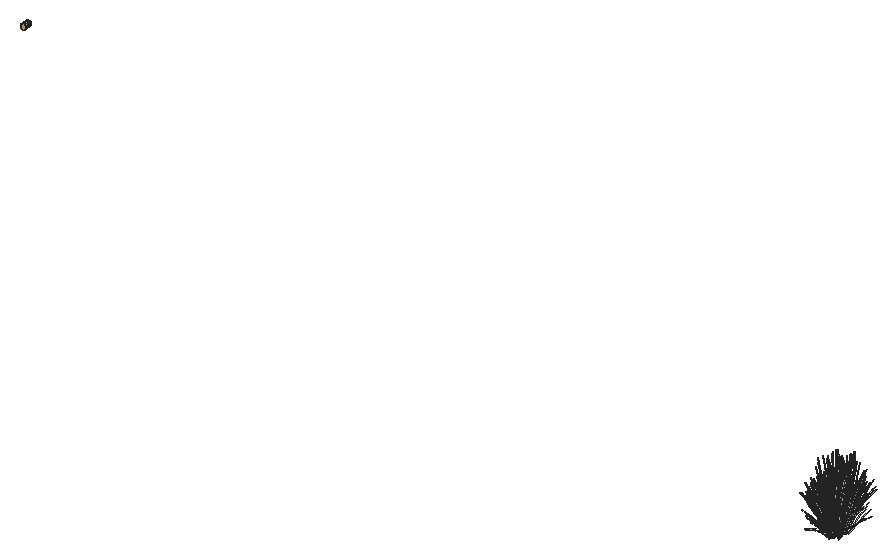
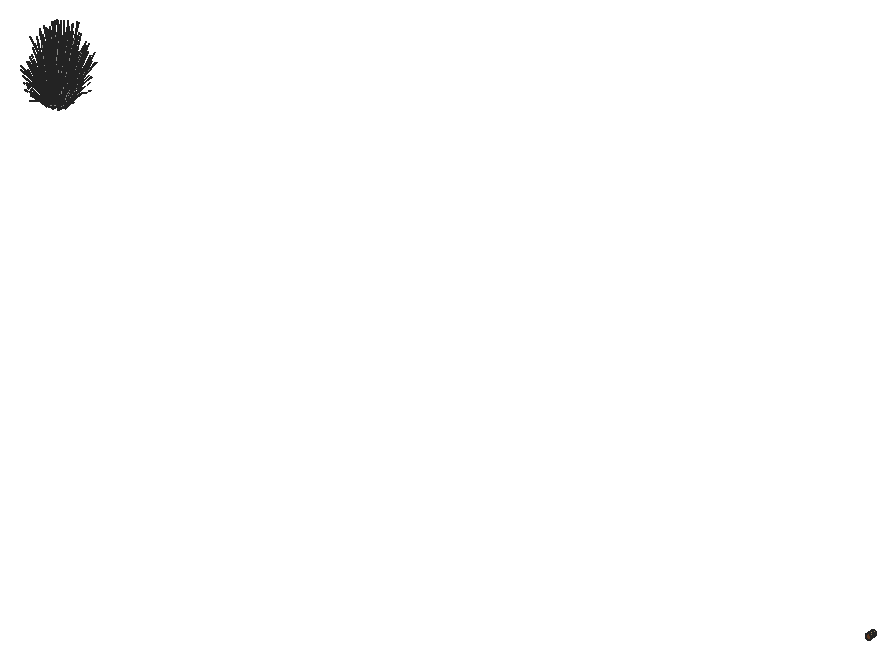
# SketchUp Ruby script. Lengths in inches.
U = 1.inch
M = Sketchup.active_model
def pt(a) = Geom::Point3d.new(a.map { |v| v * U })
def face(e, loops, mat)
  f = e.add_face(loops[0].map { |a| pt(a) })
  loops[1..].each { |l| e.add_face(l.map { |a| pt(a) }).erase! }
  f.material = f.back_material = mat if mat
  f
end
# faces: each face lists its corners as indices into pts; further lists are holes
def faces(e, pts, list, mat = nil) = list.each { |f| face(e, (f[0].is_a?(Array) ? f : [f]).map { |l| l.map { |i| pts[i] } }, mat) }
# xy, xz, yz: faces in a plane at the given z, y or x. An outline is a flat list of corners, or four numbers for a rectangle; further outlines are holes
def ring(l) = l.size == 4 ? [[l[0], l[1]], [l[2], l[1]], [l[2], l[3]], [l[0], l[3]]] : l.each_slice(2).to_a
def flat(e, list, mat, &to3) = list.each { |f| face(e, (f[0].is_a?(Array) ? f : [f]).map { |l| ring(l).map { |u, v| to3.(u, v) } }, mat) }
def xy(e, z, list, mat = nil) = flat(e, list, mat) { |x, y| [x, y, z] }
def xz(e, y, list, mat = nil) = flat(e, list, mat) { |x, z| [x, y, z] }
def yz(e, x, list, mat = nil) = flat(e, list, mat) { |y, z| [x, y, z] }
def lines(e, pts, list) = list.each { |a, b| e.add_line(pt(pts[a]), pt(pts[b])) }
# prism: a flat outline (further loops are holes) pulled along v
def prism(e, loops, v, mat = nil)
  f = face(e, loops, mat); d = Geom::Vector3d.new(v.map { |x| x * U })
  f.pushpull(f.normal.samedirection?(d) ? d.length : -d.length)
end
def box(e, o, s, mat = nil) = prism(e, [[o, [o[0] + s[0], o[1], o[2]], [o[0] + s[0], o[1] + s[1], o[2]], [o[0], o[1] + s[1], o[2]]]], [0, 0, s[2]], mat)
def at(x, y, z, deg = 0) = Geom::Transformation.translation(pt([x, y, z])) * Geom::Transformation.rotation(ORIGIN, Z_AXIS, deg.degrees)
def axes(o, x, y, z) = Geom::Transformation.new([*x, 0, *y, 0, *z, 0, *pt(o).to_a, 1])
def part(name) = M.definitions.add(name)
# library, detail: a bought-in or finely detailed component or shape, given as its bounding box
def library(name, o, s) = part(name).tap { |d| box(d.entities, o, s) }
def detail(e, o, s) = box(e.add_group.entities, o, s)
def put(e, d, t, mat = nil) = e.add_instance(d, t).tap { |i| i.material = mat if mat }
def group(e, t, mat = nil) = e.add_group.tap { |g| g.transformation = t; g.material = mat if mat }.entities
root = M.entities
M.materials.add("[Wood Cherry Original]").color = [152, 86, 42]
M.materials.add("[Wood Floor Light]").color = [204, 176, 127]
c1 = part("blade")
p = [[2.15,0.21,22],[0,0.17,0],[0.09,0.45,0],[2.18,0.31,22],[2.29,0.31,22],[0.38,0.45,0],
  [2.48,0.24,33],[2.49,0.24,33],[2.48,0.22,33]]
faces(c1.entities,p,[[0,1,2,3],[4,5,2,3],[6,3,4,7],[8,0,3,6]])
c2 = part("blade with seeds\#1")
put(c2.entities,c1,at(0,0,0))
xz(root,239.125,[[277.8,222.23,278.32,222.3,278.8,222.5,279.21,222.8125,279.53,223.23,279.73,223.71,279.8,224.23,279.73,224.74,279.53,225.23,279.21,225.64,278.8,225.96,278.32,226.16,277.8,226.23,277.28,226.16,276.8,225.96,276.38,225.64,276.07,225.23,275.87,224.74,275.8,224.23,275.87,223.71,276.07,223.23,276.38,222.8125,276.8,222.5,277.28,222.3]],"[Wood Floor Light]")
xz(root,244.125,[[277.8,222.23,277.28,222.3,276.8,222.5,276.38,222.8125,276.07,223.23,275.87,223.71,275.8,224.23,275.87,224.74,276.07,225.23,276.38,225.64,276.8,225.96,277.28,226.16,277.8,226.23,278.32,226.16,278.8,225.96,279.21,225.64,279.53,225.23,279.73,224.74,279.8,224.23,279.73,223.71,279.53,223.23,279.21,222.8125,278.8,222.5,278.32,222.3]],"[Wood Cherry Original]")
p = [[277.28,244.125,222.3],[277.8,244.125,222.23],[277.8,239.125,222.23],[277.28,239.125,222.3],[278.32,244.125,222.3],[278.32,239.125,222.3],
  [276.8,244.125,222.5],[276.8,239.125,222.5],[278.8,244.125,222.5],[278.8,239.125,222.5],[276.38,244.125,222.8125],[276.38,239.125,222.8125],
  [279.21,244.125,222.8125],[279.21,239.125,222.8125],[276.07,244.125,223.23],[276.07,239.125,223.23],[279.53,244.125,223.23],[279.53,239.125,223.23],
  [275.87,244.125,223.71],[275.87,239.125,223.71],[279.73,244.125,223.71],[279.73,239.125,223.71],[275.8,244.125,224.23],[275.8,239.125,224.23],
  [279.8,244.125,224.23],[279.8,239.125,224.23],[275.87,244.125,224.74],[275.87,239.125,224.74],[279.73,244.125,224.74],[279.73,239.125,224.74],
  [276.07,244.125,225.23],[276.07,239.125,225.23],[279.53,244.125,225.23],[279.53,239.125,225.23],[276.38,244.125,225.64],[276.38,239.125,225.64],
  [279.21,244.125,225.64],[279.21,239.125,225.64],[276.8,244.125,225.96],[276.8,239.125,225.96],[278.8,244.125,225.96],[278.8,239.125,225.96],
  [277.28,244.125,226.16],[277.28,239.125,226.16],[278.32,244.125,226.16],[278.32,239.125,226.16],[277.8,244.125,226.23],[277.8,239.125,226.23],
  [277.8,244.125,224.23],[277.8,239.125,224.23]]
faces(root,p,[[0,1,2,3],[1,4,5,2],[6,0,3,7],[4,8,9,5],[10,6,7,11],[8,12,13,9],[14,10,11,15],[12,16,17,13],
  [18,14,15,19],[16,20,21,17],[22,18,19,23],[20,24,25,21],[26,22,23,27],[24,28,29,25],[30,26,27,31],[28,32,33,29],
  [34,30,31,35],[32,36,37,33],[38,34,35,39],[36,40,41,37],[42,38,39,43],[40,44,45,41],[46,42,43,47],[44,46,47,45]],"[Wood Floor Light]")
lines(root,p,[[48,49]])
put(root,c2,axes([1022.19,59.2,233.03],[0.31369,-0.26428,1.54493],[0.26409,1.22118,0.12492],[-0.49247,0.276,0.66044]))
put(root,c2,axes([1020.11,57.1875,233.79],[-0.13699,0.17683,1.57709],[0.08685,1.18009,-0.24942],[-0.32765,0.18834,0.12648]))
put(root,c2,axes([1021.74,54.45,231.87],[0.19776,0.32863,1.28914],[-0.34614,0.98419,-0.27724],[-0.43048,-0.18244,0.55117]))
put(root,c2,axes([1022.42,55.95,234.03],[-0.79444,0.5518,-0.64046],[-0.44274,-1.13586,0.07729],[-0.38385,0.12903,0.906]))
put(root,c2,axes([1021.36,59.54,231.87],[0.31962,0.07001,1.28914],[0.26756,1.02347,-0.27724],[-0.41311,0.23924,0.55117]))
put(root,c2,axes([1020.66,56.9,230.88],[0.0352,0.19392,1.5897],[-0.39624,1.07238,-0.24285],[-0.33051,-0.01799,0.27078]))
put(root,c2,axes([1021.09,52.14,233.78],[0.07463,0.11741,1.59908],[-0.25178,1.15035,-0.1511],[-0.32567,0.04164,0.28298]))
put(root,c2,axes([1021.79,51.88,233.79],[-0.19445,0.01116,1.57709],[-0.562,0.94258,-0.24942],[-0.34067,-0.14573,0.12648]))
put(root,c2,axes([1023.2,53.65,234.03],[-0.90375,-0.03008,-0.64046],[0.0607,-1.26677,0.07729],[-0.38287,-0.13368,0.906]))
put(root,c2,axes([1022.74,55.08,233.03],[0.33582,0.21526,1.54493],[-0.69497,0.90306,0.12492],[-0.43315,-0.40739,0.66044]))
put(root,c2,axes([1021.75,55.84,233.62],[-0.75135,-0.34854,-0.31925],[0.21915,-1.01686,0.41216],[-0.30251,0.09324,0.78863]))
put(root,c2,axes([1020.16,55.66,232.03],[0.56973,-0.14831,1.03545],[-0.31555,0.82274,0.76078],[-0.29172,-0.08853,0.22807]))
put(root,c2,axes([1022.26,56.36,233.76],[-0.24493,1.13649,-0.46065],[-0.83975,-0.38955,-0.35681],[-0.33809,0.10421,0.88141]))
put(root,c2,axes([1019.66,58.4,233.78],[0.11711,0.02157,1.59908],[0.42502,1.06376,-0.1511],[-0.21726,0.31303,0.28298]))
put(root,c2,axes([1022.9,53.91,233.76],[-0.65648,0.82762,-0.46065],[-0.57493,-0.87428,-0.35681],[-0.33354,-0.12593,0.88141]))
put(root,c2,axes([1022.22,55.39,234.08],[0.45489,1.13134,-0.10962],[-0.80735,0.55596,-0.60845],[-0.34022,0.14927,0.92453]))
put(root,c2,axes([1021.74,58.63,234.13],[-0.25113,-1.28788,0.48466],[0.9851,-0.22351,0.39963],[-0.29033,0.30289,1.00289]))
put(root,c2,axes([1020.85,59.89,232.03],[0.34005,-0.60308,1.03545],[0.20441,0.87829,0.76078],[-0.26134,0.18792,0.22807]))
put(root,c2,axes([1021.92,55.72,233.8],[0.25543,-1.1392,0.43274],[0.83975,0.38955,0.35681],[-0.33023,0.06846,0.89544]))
put(root,c2,axes([1023.25,53.04,234.08],[-0.04841,1.27062,-0.10962],[-0.91657,-0.03473,-0.60845],[-0.353,-0.08826,0.92453]))
put(root,c2,axes([1022.65,58.43,234.03],[-0.47225,0.98582,-0.64046],[-0.82754,-0.7006,0.07729],[-0.28197,0.35717,0.906]))
put(root,c2,axes([1021.86,55.42,233.8],[-0.33205,-0.8519,0.05797],[0.60551,-0.41697,0.45634],[-0.26692,0.08227,0.69585]))
put(root,c2,axes([1022.02,58.78,233.62],[-0.78697,0.17856,-0.31925],[-0.2078,-1.02074,0.41216],[-0.22552,0.27417,0.78863]))
put(root,c2,axes([1022.66,53.13,233.62],[-0.51441,-0.78225,-0.31925],[0.58738,-0.7405,0.41216],[-0.29843,-0.11267,0.78863]))
put(root,c2,axes([1021.87,60.37,230.88],[0.12871,0.11199,1.5897],[0.2775,1.13173,-0.24285],[-0.25244,0.2734,0.27078]))
put(root,c2,axes([1021.95,58.33,233.8],[-0.62066,-0.52545,0.05797],[0.36135,-0.74826,0.45634],[-0.19899,0.24191,0.69585]))
put(root,c2,axes([1022.35,52.15,230.88],[-0.07697,0.17304,1.5897],[-0.85991,0.44448,-0.24285],[-0.23336,-0.29985,0.27078]))
put(root,c2,axes([1023.17,60.97,233.03],[0.16834,-0.42944,1.54493],[0.70619,0.88871,0.12492],[-0.31858,0.5539,0.66044]))
put(root,c2,axes([1022.54,55.73,234.09],[0.75135,0.34854,0.31925],[-0.21915,1.01686,-0.41216],[-0.30251,0.09324,0.78863]))
put(root,c2,axes([1025.41,58.5,231.43],[-1.0019,0.47479,-0.62955],[-0.36083,-1.36768,-0.16523],[-0.33927,0.05248,1.38963]))
put(root,c2,axes([1021.89,58.1,234.43],[0.93666,0.77159,-0.12278],[-0.53962,1.11741,-0.68147],[-0.26463,0.38842,1.03548]))
put(root,c2,axes([1022.67,58.9,233.76],[0.23225,1.14083,-0.46065],[-0.87956,0.19957,-0.35681],[-0.25205,0.30642,0.88141]))
put(root,c2,axes([1022.86,53.13,233.8],[0.66663,-0.82326,0.43274],[0.57493,0.87428,0.35681],[-0.31276,-0.15186,0.89544]))
put(root,c2,axes([1022.92,52.83,233.8],[0.04552,-0.95007,0.05797],[0.68742,0.02605,0.45634],[-0.26332,-0.09941,0.69585]))
put(root,c2,axes([1023.39,53.54,234.09],[0.51441,0.78225,0.31925],[-0.58738,0.7405,-0.41216],[-0.29843,-0.11267,0.78863]))
put(root,c2,axes([1021.35,57.1,231.46],[0.56051,0.79893,-0.03509],[-0.61388,0.73204,-0.15911],[-0.17394,0.05154,0.52479]))
put(root,c2,axes([1022.53,58.6875,231.68],[-0.97904,0.72283,0],[-0.54599,-1.20931,-0.46523],[-0.12435,-0.27543,1.47583]))
put(root,c2,axes([1024.41,52.1875,233.76],[-0.89213,0.297,-0.46065],[-0.15606,-1.12475,-0.35681],[-0.23962,-0.32232,0.88141]))
put(root,c2,axes([1024.77,52.16,234.03],[-0.77091,-0.6039,-0.64046],[0.54787,-1.05824,0.07729],[-0.27931,-0.36058,0.906]))
put(root,c2,axes([1021.62,61.06,233.79],[-0.0069,0.24875,1.57709],[0.68965,0.79195,-0.24942],[-0.14092,0.42256,0.12648]))
put(root,c2,axes([1025.05,51.66,234.08],[-0.53874,1.06944,-0.10962],[-0.78019,-0.61612,-0.60845],[-0.2712,-0.30214,0.92453]))
put(root,c2,axes([1022.67,58.17,234.09],[0.78697,-0.17856,0.31925],[0.2078,1.02074,-0.41216],[-0.22552,0.27417,0.78863]))
put(root,c2,axes([1024.0625,51.28,231.87],[-0.02894,0.41302,1.28914],[-0.77632,0.42312,-0.27724],[-0.21961,-0.50739,0.55117]))
put(root,c2,axes([1022.375,57.7,231.36],[-0.48852,-1.08202,-0.44759],[0.87598,-0.64674,0],[-0.11126,-0.24644,1.41987]))
put(root,c2,axes([1024.82,49.02,233.78],[-0.00742,0.151,1.59908],[-0.79509,0.62706,-0.1511],[-0.26143,-0.25182,0.28298]))
put(root,c2,axes([1022.64,50.81,232.03],[0.49736,0.38508,1.03545],[-0.66822,0.331,0.76078],[-0.16744,-0.31805,0.22807]))
put(root,c2,axes([1023.18,61.24,234.13],[-0.72104,-0.95477,0.48466],[0.76573,-0.82343,0.39963],[-0.133,0.44794,1.00289]))
put(root,c2,axes([1025.27,61.3,231.36],[-0.97703,0,-0.44759],[0,-1.29348,0],[-0.22253,0,1.41987]))
put(root,c2,axes([1027.99,56.07,232.53],[0.39398,-0.99907,1.36359],[0.84877,0.97875,0.53923],[-0.50305,0.4384,1.14314]))
put(root,c2,axes([1024.38,56.42,231.39],[-0.73437,-0.77871,-0.5621],[0.66591,-0.96736,-0.14753],[-0.18319,-0.31204,1.24074]))
put(root,c2,axes([1023.17,60.8,233.8],[-0.74296,-0.05822,0.05797],[0.02037,-0.87906,0.45634],[-0.07774,0.33673,0.69585]))
put(root,c2,axes([1023.41,61.14,233.62],[-0.61172,0.65782,-0.31925],[-0.57907,-0.75112,0.41216],[-0.08811,0.38163,0.78863]))
put(root,c2,axes([1024.51,51.36,233.62],[-0.13963,-1.00636,-0.31925],[0.79822,-0.26574,0.41216],[-0.2144,-0.28839,0.78863]))
put(root,c2,axes([1022.37,61.07,231.46],[0.7978,0.33351,-0.03509],[-0.24541,1.02647,-0.15911],[-0.13049,0.15585,0.52479]))
put(root,c2,axes([1025.67,57.78,231.53],[-0.88038,-0.56093,-0.40331],[0.4237,-1.16553,0.1941],[-0.20294,0,1.29492]))
put(root,c2,axes([1024.98,52.18,234.09],[0.13963,1.00636,0.31925],[-0.79822,0.26574,-0.41216],[-0.2144,-0.28839,0.78863]))
put(root,c2,axes([1025.23,57.27,231.94],[-1.11485,0.13472,-0.26229],[-0.06741,-1.40314,-0.45076],[-0.1485,-0.24708,1.43974]))
put(root,c2,axes([1025.29,60.74,231.37],[-0.60959,-0.80703,-0.27926],[0.60959,-0.80703,0.27926],[-0.19635,0,1.25283]))
put(root,c2,axes([1026.4,57.92,231.94],[-0.46619,1.302,-0.26229],[-0.98396,-0.62692,-0.45076],[-0.24158,0.04092,1.43974]))
put(root,c2,axes([1026.01,61.62,231.68],[0,1.44565,0],[-1.09198,0,-0.46523],[-0.24871,0,1.47583]))
put(root,c2,axes([1022.76,57.45,231.37],[0.24175,-1.0786,-0.27926],[0.85134,0.27158,0.27926],[-0.09817,-0.21744,1.25283]))
put(root,c2,axes([1024.06,61.375,231.87],[0.27202,-0.22572,1.28914],[0.7394,0.52014,-0.27724],[-0.17673,0.53408,0.55117]))
put(root,c2,axes([1023.82,60.44,234.03],[-0.02352,1.1557,-0.64046],[-0.99061,-0.07762,0.07729],[-0.10454,0.48961,0.906]))
put(root,c2,axes([1024.68,51.49,233.8],[0.89921,-0.28673,0.43274],[0.15606,1.12475,0.35681],[-0.21148,-0.33149,0.89544]))
put(root,c2,axes([1024.85,51.27,233.8],[0.4109,-0.79368,0.05797],[0.58514,0.46209,0.45634],[-0.18917,-0.25446,0.69585]))
put(root,c2,axes([1025.77,48.46,233.79],[-0.14882,-0.16043,1.57709],[-0.91289,0.20534,-0.24942],[-0.17308,-0.40254,0.12648]))
put(root,c2,axes([1025.72,60.5,231.64],[0.82143,1.07538,0.27726],[-0.81279,1.07603,-0.32897],[-0.23327,0.03755,1.48641]))
put(root,c2,axes([1022.2,62.01,233.78],[0.0975,-0.08571,1.59908],[0.87648,0.41319,-0.1511],[0.00634,0.41846,0.28298]))
put(root,c2,axes([1024.02,60.83,233.76],[0.6472,0.83949,-0.46065],[-0.68369,0.73521,-0.35681],[-0.09847,0.42653,0.88141]))
put(root,c2,axes([1023.73,60.21,234.09],[0.61172,-0.65782,0.31925],[0.57907,0.75112,-0.41216],[-0.08811,0.38163,0.78863]))
put(root,c2,axes([1026.1,57.08,231.73],[0.47355,-1.30265,0.21694],[0.98396,0.62692,0.45076],[-0.22682,0,1.44726]))
put(root,c2,axes([1027.43,57.59,231.74],[-1.15773,-0.30643,-0.21121],[0.20181,-1.4529,0.4622],[-0.15988,0.25387,1.41028]))
put(root,c2,axes([1023.34,60.39,234.08],[0.99362,0.0619,-0.10962],[-0.02716,1.17208,-0.60845],[-0.06902,0.45141,0.92453]))
put(root,c2,axes([1024.875,62.72,232.03],[-0.06991,-0.73811,1.03545],[0.616,0.4682,0.76078],[-0.09241,0.36475,0.22807]))
put(root,c2,axes([1025.45,57.5,231.99],[0.06031,1.25545,0.40331],[-1.00118,0.11354,-0.1941],[-0.10147,-0.22475,1.29492]))
put(root,c2,axes([1026.18,60.74,231.77],[0.97703,0,0.44759],[0,1.29348,0],[-0.22253,0,1.41987]))
put(root,c2,axes([1022.77,53.36,231.68],[-0.97904,-0.72283,0],[0.54599,-1.20931,-0.46523],[0.12435,-0.27543,1.47583]))
put(root,c2,axes([1025.81,57.55,231.67],[1.09253,-0.50265,0.41247],[0.37991,1.43622,0.16186],[-0.20075,-0.01755,1.43206]))
put(root,c2,axes([1027.15,51.61,234.08],[-0.88471,0.5817,-0.10962],[-0.43476,-1.03242,-0.60845],[-0.11673,-0.43507,0.92453]))
put(root,c2,axes([1024.71,61.88,233.03],[-0.02213,-0.47954,1.54493],[0.95907,0.31812,0.12492],[-0.05932,0.68338,0.66044]))
put(root,c2,axes([1026.39,51.67,233.76],[-0.88873,-0.31321,-0.46065],[0.30463,-1.07385,-0.35681],[-0.08149,-0.43235,0.88141]))
put(root,c2,axes([1026.96,57.69,231.53],[-0.82007,0.69452,-0.40331],[-0.57748,-1.05199,0.1941],[-0.10147,0.22475,1.29492]))
put(root,c2,axes([1026.64,50.52,231.32],[0.11725,0.74462,1.27635],[-0.9333,0.11852,0.07306],[-0.14126,-0.52153,0.72629]))
put(root,c2,axes([1025.82,49.16,231.57],[-0.62476,0.71677,-0.05849],[-0.57245,-0.78502,-0.26518],[-0.0403,-0.22243,0.87466]))
put(root,c2,axes([1023.29,53.99,231.77],[-0.48852,1.08202,0.44759],[-0.87598,-0.64674,0],[0.11126,-0.24644,1.41987]))
put(root,c2,axes([1026.67,57.8,231.99],[0.88038,0.56093,0.40331],[-0.4237,1.16553,-0.1941],[-0.20294,0,1.29492]))
put(root,c2,axes([1025.9,55.74,231.52],[-1.1305,0,0],[0,-1.44565,0],[0,0,1.61777]))
put(root,c2,axes([1025.1875,56.42,231.67],[0.88667,0.95859,0.41247],[-0.7827,1.13884,0.16186],[-0.08849,-0.2311,1.43206]))
put(root,c2,axes([1023.73,58.09,231.77],[0.971,0.33398,0.15904],[-0.27478,1.22215,0.3163],[-0.00473,-0.21112,1.44604]))
put(root,c2,axes([1026.72,51.87,234.03],[-0.4315,-1.0159,-0.64046],[0.88824,-0.56616,0.07729],[-0.1009,-0.49086,0.906]))
put(root,c2,axes([1027.28,58.3125,231.39],[-0.16018,1.20264,-0.5621],[-0.98808,-0.25378,-0.14753],[-0.11973,0.3589,1.24074]))
put(root,c2,axes([1024.51,58.59,230.97],[0.39117,1.13797,1.16227],[-1.12236,0.3622,0.45161],[0.01867,-0.69878,1.32195]))
put(root,c2,axes([1026.77,55.375,231.61],[-0.84094,1.07538,-0.05527],[-0.84146,-1.07603,0],[-0.02937,0.03755,1.58274]))
put(root,c2,axes([1026.89,52.02,234.09],[-0.27256,0.96081,0.31925],[-0.79518,-0.28024,-0.41216],[-0.07291,-0.38684,0.78863]))
put(root,c2,axes([1024.81,55.54,231.9],[-0.87196,-0.22303,0.13053],[0.15136,-1.08968,-0.37274],[0.08953,-0.19831,1.14258]))
put(root,c2,axes([1025.43,62.08,233.8],[-0.89085,-0.32663,0.43274],[0.30463,-1.07385,0.35681],[0.05354,0.4223,0.89544]))
put(root,c2,axes([1025.2,62.16,233.8],[-0.66618,0.42462,0.05797],[-0.32607,-0.77431,0.45634],[0.06434,0.34133,0.69585]))
put(root,c2,axes([1026.03,49.71,230.88],[-0.14833,0.06042,1.5897],[-0.86768,-0.41907,-0.24285],[-0.01248,-0.42273,0.27078]))
put(root,c2,axes([1025.04,56,231.99],[-0.82007,0.69452,0.40331],[-0.57748,-1.05199,-0.1941],[0.10147,-0.22475,1.29492]))
put(root,c2,axes([1026.875,57.42,231.67],[0.20585,-1.46124,0.41247],[1.16261,0.29738,0.16186],[-0.11226,0.21355,1.43206]))
put(root,c2,axes([1025.88,62.18,230.88],[0.15398,-0.02932,1.5897],[0.80412,0.59108,-0.24285],[-0.04053,0.41985,0.27078]))
put(root,c2,axes([1028.78,59.59,231.37],[-0.85134,0.27158,-0.27926],[-0.24175,-1.0786,0.27926],[-0.09817,0.21744,1.25283]))
put(root,c2,axes([1023.36,52.7,231.36],[0.48852,-1.08202,-0.44759],[0.87598,0.64674,0],[0.11126,-0.24644,1.41987]))
put(root,c2,axes([1025.09,55.65,231.94],[-0.64866,-1.16728,-0.26229],[0.91655,-0.77622,-0.45076],[0.09308,-0.288,1.43974]))
put(root,c2,axes([1023.78,54.39,231.77],[0.25932,1.24233,0.15904],[-0.96507,0.30677,0.3163],[0.14061,-0.1108,1.44604]))
put(root,c2,axes([1025.53,62.3,233.62],[-0.27256,0.96081,-0.31925],[-0.79518,-0.28024,0.41216],[0.07291,0.38684,0.78863]))
put(root,c2,axes([1026.8,51.01,233.62],[0.27256,-0.96081,-0.31925],[0.79518,0.28024,0.41216],[-0.07291,-0.38684,0.78863]))
put(root,c2,axes([1028.73,58.21,231.77],[-0.25932,-1.24233,0.15904],[0.96507,-0.30677,0.3163],[-0.14061,0.1108,1.44604]))
put(root,c2,axes([1027.42,56.95,231.94],[0.64866,1.16728,-0.26229],[-0.91655,0.77622,-0.45076],[-0.09308,0.288,1.43974]))
put(root,c2,axes([1029.15,59.89,231.36],[-0.48852,1.08202,-0.44759],[-0.87598,-0.64674,0],[-0.11126,0.24644,1.41987]))
put(root,c2,axes([1026.15,54.76,231.53],[0,-1.29348,0],[1.0115,0,0],[0,0,1.60831]))
put(root,c2,axes([1023.73,53.01,231.37],[0.85134,-0.27158,-0.27926],[0.24175,1.0786,0.27926],[0.09817,-0.21744,1.25283]))
put(root,c2,axes([1025.81,53.625,233.03],[0.02213,0.47954,1.54493],[-0.95907,-0.31812,0.12492],[0.05932,-0.68338,0.66044]))
put(root,c2,axes([1025.64,55.18,231.68],[-0.20585,1.46124,0.44352],[-1.16261,-0.29738,0.17404],[0.11226,-0.21355,1.53985]))
put(root,c2,axes([1027.13,51.15,233.8],[0.66618,-0.42462,0.05797],[0.32607,0.77431,0.45634],[-0.06434,-0.34133,0.69585]))
put(root,c2,axes([1026.9,51.23,233.8],[0.89085,0.32663,0.43274],[-0.30463,1.07385,0.35681],[-0.05354,-0.4223,0.89544]))
put(root,c2,axes([1025.44,61.29,234.09],[0.27256,-0.96081,0.31925],[0.79518,0.28024,-0.41216],[0.07291,0.38684,0.78863]))
put(root,c2,axes([1027.71,57.0625,231.9],[0.87196,0.22303,0.13053],[-0.15136,1.08968,-0.37274],[-0.08953,0.19831,1.14258]))
put(root,c2,axes([1028.51,56.34,231.52],[-0.84234,0.37722,0],[-0.29498,-1.07717,0],[0,0,1.39163]))
put(root,c2,axes([1026.59,54.79,231.53],[0.63109,-0.80703,0],[0.63109,0.80703,0],[0,0,1.52591]))
put(root,c2,axes([1026.31,52.6,231.77],[-0.71168,0.90835,0.15904],[-0.69029,-0.91538,0.3163],[0.14534,0.10032,1.44604]))
put(root,c2,axes([1028.39,54.93,231.51],[-0.33151,-1.21377,-0.17307],[0.95493,-0.4265,0.00007],[-0.03664,-0.13398,1.56765]))
put(root,c2,axes([1025.4,59.375,232.55],[-0.14134,-0.32863,1.5962],[0.98684,-0.11332,0.12492],[0.13095,0.71181,0.57049]))
put(root,c2,axes([1026.96,48.97,232.03],[0.1613,0.71432,1.03545],[-0.66662,-0.33623,0.76078],[0.04561,-0.37895,0.22807]))
put(root,c2,axes([1025.23,54.28,231.39],[0.16018,-1.20264,-0.5621],[0.98808,0.25378,-0.14753],[0.11973,-0.3589,1.24074]))
put(root,c2,axes([1028.79,54.51,231.77],[-0.971,-0.33398,0.15904],[0.27478,-1.22215,0.3163],[0.00473,0.21112,1.44604]))
put(root,c2,axes([1027.72,55.64,231.76],[-0.78639,1.12892,-0.2271],[-0.88305,-0.94994,0.49699],[0.09199,0.304,1.51643]))
put(root,c2,axes([1028.89,56.61,231.52],[-0.43865,1.16553,0],[-0.91144,-0.56093,0],[0,0,1.46678]))
put(root,c2,axes([1025.85,54.8,231.99],[-0.88038,-0.56093,0.40331],[0.4237,-1.16553,-0.1941],[0.20294,0,1.29492]))
put(root,c2,axes([1029.23,58.61,231.77],[0.48852,-1.08202,0.44759],[0.87598,0.64674,0],[-0.11126,0.24644,1.41987]))
put(root,c2,axes([1025.9375,61.64,233.76],[0.88873,0.31321,-0.46065],[-0.30463,1.07385,-0.35681],[0.08149,0.43235,0.88141]))
put(root,c2,axes([1025.18,61.69,234.08],[0.88471,-0.5817,-0.10962],[0.43476,1.03242,-0.60845],[0.11673,0.43507,0.92453]))
put(root,c2,axes([1026.35,55.01,231.6],[1.12994,0,-0.05082],[0,1.44565,0],[0.03551,0,1.61697]))
put(root,c2,axes([1029.78,49.3,233.78],[-0.08553,0.10454,1.59908],[-0.91687,-0.22868,-0.1511],[-0.05858,-0.41178,0.28298]))
put(root,c2,axes([1025.55,54.91,231.53],[0.82007,-0.69452,-0.40331],[0.57748,1.05199,0.1941],[0.10147,-0.22475,1.29492]))
put(root,c2,axes([1026.0625,62.91,233.79],[0.12685,0.18879,1.57709],[0.92682,-0.01606,-0.24942],[0.12053,0.43275,0.12648]))
put(root,c2,axes([1029.74,59.23,231.68],[0.97904,0.72283,0],[-0.54599,1.20931,-0.46523],[-0.12435,0.27543,1.47583]))
put(root,c2,axes([1026.34,51.85,231.77],[-0.97703,0,0.44759],[0,-1.29348,0],[0.22253,0,1.41987]))
put(root,c2,axes([1029.02,50.21,233.08],[-0.82131,0.22128,-0.03148],[-0.18882,-1.04586,-0.14272],[0.05207,-0.2184,0.47074]))
put(root,c2,axes([1028.99,52.92,234.08],[-0.99362,-0.0619,-0.10962],[0.02716,-1.17208,-0.60845],[0.06902,-0.45141,0.92453]))
put(root,c2,axes([1026.05,54.31,231.9],[-0.28493,-1.07717,0.13053],[0.81364,-0.37722,-0.37274],[0.17907,0,1.14258]))
put(root,c2,axes([1027.07,55.09,231.99],[-0.06031,-1.25545,0.40331],[1.00118,-0.11354,-0.1941],[0.10147,0.22475,1.29492]))
put(root,c2,axes([1027.55,56.21,231.53],[0.06031,1.25545,-0.40331],[-1.00118,0.11354,0.1941],[0.10147,0.22475,1.29492]))
put(root,c2,axes([1028.6,53.1,234.09],[-0.61172,0.65782,0.31925],[-0.57907,-0.75112,-0.41216],[0.08811,-0.38163,0.78863]))
put(root,c2,axes([1028.03,50.31,231.87],[-0.2403,0.27843,1.28914],[-0.79492,-0.36227,-0.27724],[0.10768,-0.56334,0.55117]))
put(root,c2,axes([1028.9,55.28,231.52],[0.43865,-1.16553,0],[0.91144,0.56093,0],[0,0,1.57718]))
put(root,c2,axes([1028.4,51.9,233.79],[-0.01652,-0.24801,1.57709],[-0.75906,-0.68026,-0.24942],[0.1002,-0.44114,0.12648]))
put(root,c2,axes([1027.48,62.04,233.8],[-0.4109,0.79368,0.05797],[-0.58514,-0.46209,0.45634],[0.18917,0.25446,0.69585]))
put(root,c2,axes([1027.5,55.07,231.9],[0.58702,-0.85413,0.13053],[0.66228,0.71246,-0.37274],[0.08953,0.19831,1.14258]))
put(root,c2,axes([1027.65,61.82,233.8],[-0.89921,0.28673,0.43274],[-0.15606,-1.12475,0.35681],[0.21148,0.33149,0.89544]))
put(root,c2,axes([1026.4,61.68,233.03],[-0.20666,-0.40114,1.54493],[0.95496,-0.33772,0.12492],[0.21583,0.62976,0.66044]))
put(root,c2,axes([1029.875,54.82,231.51],[-0.98246,0.71382,-0.04636],[-0.54599,-1.20931,0.46523],[0.09354,0.298,1.4751]))
put(root,c2,axes([1028.51,52.86,234.03],[0.02352,-1.1557,-0.64046],[0.99061,0.07762,0.07729],[0.10454,-0.48961,0.906]))
put(root,c2,axes([1028.54,55.7,231.6],[1.12244,-0.50265,-0.0542],[0.39331,1.43622,0],[0.0392,-0.01755,1.55211]))
put(root,c2,axes([1029.75,55.15,231.37],[-0.24175,1.0786,-0.27926],[-0.85134,-0.27158,0.27926],[0.09817,0.21744,1.25283]))
put(root,c2,axes([1029.31,54.16,231.77],[-0.48852,-1.08202,0.44759],[0.87598,-0.64674,0],[0.11126,0.24644,1.41987]))
put(root,c2,axes([1027.0625,51.55,231.52],[-0.00781,1.44494,-0.04486],[-1.09198,0,0.45022],[0.24858,0.04541,1.42752]))
put(root,c2,axes([1028.02,62.93,231.87],[0.08021,-0.40179,1.28914],[0.81924,-0.25896,-0.27724],[0.15335,0.54576,0.55117]))
put(root,c2,axes([1026.5,50.97,231.68],[0,-1.44565,0],[1.09198,0,-0.46523],[0.24871,0,1.47583]))
put(root,c2,axes([1027.35,61.13,234.09],[-0.13963,-1.00636,0.31925],[0.79822,-0.26574,-0.41216],[0.2144,0.28839,0.78863]))
put(root,c2,axes([1026.11,54.68,231.94],[0.46619,-1.302,-0.26229],[0.98396,0.62692,-0.45076],[0.24158,-0.04092,1.43974]))
put(root,c2,axes([1027.22,51.85,231.37],[0.60959,0.80703,-0.27926],[-0.60959,0.80703,0.27926],[0.19635,0,1.25283]))
put(root,c2,axes([1027,65,233.78],[0.0262,-0.14755,1.59908],[0.86326,-0.45644,-0.1511],[0.22658,0.30203,0.28298]))
put(root,c2,axes([1027.28,55.33,231.94],[1.11485,-0.13472,-0.26229],[0.06741,1.40314,-0.45076],[0.1485,0.24708,1.43974]))
put(root,c2,axes([1026.85,54.82,231.53],[0.88038,0.56093,-0.40331],[-0.4237,1.16553,0.1941],[0.20294,0,1.29492]))
put(root,c2,axes([1027.83,61.95,233.62],[0.13963,1.00636,-0.31925],[-0.79822,0.26574,0.41216],[0.2144,0.28839,0.78863]))
put(root,c2,axes([1028.92,52.17,233.62],[0.61172,-0.65782,-0.31925],[0.57907,0.75112,0.41216],[0.08811,-0.38163,0.78863]))
put(root,c2,axes([1029.16,52.5,233.8],[0.74296,0.05822,0.05797],[-0.02037,0.87906,0.45634],[0.07774,-0.33673,0.69585]))
put(root,c2,axes([1028.92,52.42,233.8],[0.64379,0.85247,0.43274],[-0.68369,0.73521,0.35681],[0.11875,-0.39995,0.89544]))
put(root,c2,axes([1029.74,63.77,232.03],[-0.44281,-0.48182,1.03545],[0.70101,-0.19012,0.76078],[0.12552,0.34819,0.22807]))
put(root,c2,axes([1028.13,56.17,231.39],[0.73437,0.77871,-0.5621],[-0.66591,0.96736,-0.14753],[0.18319,0.31204,1.24074]))
put(root,c2,axes([1025.14,54.45,233.57],[-0.50765,0.99901,1.24659],[-0.79039,-1.05487,0.53787],[0.47632,-0.32232,1.20495]))
put(root,c2,axes([1027.24,51.3,231.36],[0.97703,0,-0.44759],[0,1.29348,0],[0.22253,0,1.41987]))
put(root,c2,axes([1027.35,54.53,233.03],[-0.16834,0.42944,1.54493],[-0.70619,-0.88871,0.12492],[0.31858,-0.5539,0.66044]))
put(root,c2,axes([1029.62,63.41,234.625],[0.2608,-1.0202,-0.05849],[0.8027,0.31383,-0.26518],[0.12187,0.16686,0.87466]))
put(root,c2,axes([1030.14,54.89,231.36],[0.48852,1.08202,-0.44759],[-0.87598,0.64674,0],[0.11126,0.24644,1.41987]))
put(root,c2,axes([1029.66,55.13,234.09],[-0.78697,0.17856,0.31925],[-0.2078,-1.02074,-0.41216],[0.22552,-0.27417,0.78863]))
put(root,c2,axes([1029.37,54.79,231.64],[0.31757,-1.44738,0.27726],[1.13512,0.3621,-0.32897],[0.14207,0.23956,1.48641]))
put(root,c2,axes([1027.28,61.65,234.08],[0.53874,-1.06944,-0.10962],[0.78019,0.61612,-0.60845],[0.2712,0.30214,0.92453]))
put(root,c2,axes([1029.27,52.94,232.03],[-0.28093,0.65095,1.03545],[-0.28545,-0.84053,0.76078],[0.2418,-0.22671,0.22807]))
put(root,c2,axes([1027.04,60.21,233.03],[-0.3002,-0.28876,1.54493],[0.81031,-0.72911,0.12492],[0.36902,0.50009,0.66044]))
put(root,c2,axes([1027.92,61.12,233.76],[0.89213,-0.297,-0.46065],[0.15606,1.12475,-0.35681],[0.23962,0.32232,0.88141]))
put(root,c2,axes([1030.07,55.23,234.08],[-0.8363,-0.68892,-0.10962],[0.4818,-0.99769,-0.60845],[0.23628,-0.3468,0.92453]))
put(root,c2,axes([1027.11,54.16,231.43],[0.89455,-0.42392,-0.62393],[0.32217,1.22114,-0.16376],[0.30292,-0.04686,1.37722]))
put(root,c2,axes([1026.11,54.53,232.1],[-0.91991,0.03158,1.27354],[0.23846,-1.42935,0.53923],[0.50337,0.33806,1.20213]))
put(root,c2,axes([1028.94,59.77,234.09],[-0.51441,-0.78225,0.31925],[0.58738,-0.7405,-0.41216],[0.29843,0.11267,0.78863]))
put(root,c2,axes([1029.99,53.91,231.68],[0.97904,-0.72283,0],[0.54599,1.20931,-0.46523],[0.12435,0.27543,1.47583]))
put(root,c2,axes([1029.41,60.48,233.8],[-0.04552,0.95007,0.05797],[-0.68742,-0.02605,0.45634],[0.26332,0.09941,0.69585]))
put(root,c2,axes([1030.77,56.13,233.78],[-0.11829,-0.00342,1.59908],[-0.52187,-0.99076,-0.1511],[0.18628,-0.34414,0.28298]))
put(root,c2,axes([1030.3125,52.76,230.88],[-0.14106,-0.08423,1.5897],[-0.41543,-1.06044,-0.24285],[0.21501,-0.3215,0.27078]))
put(root,c2,axes([1029.47,60.18,233.8],[-0.66663,0.82326,0.43274],[-0.57493,-0.87428,0.35681],[0.31276,0.15186,0.89544]))
put(root,c2,axes([1030.19,62.5,230.88],[0.09761,-0.15508,1.5897],[0.90442,-0.26295,-0.24285],[0.19286,0.3437,0.27078]))
put(root,c2,axes([1029.66,54.41,233.76],[-0.23225,-1.14083,-0.46065],[0.87956,-0.19957,-0.35681],[0.25205,-0.30642,0.88141]))
put(root,c2,axes([1029.79,57.58,234.09],[-0.75135,-0.34854,0.31925],[0.21915,-1.01686,-0.41216],[0.30251,-0.09324,0.78863]))
put(root,c2,axes([1030.55,52.84,231.94],[-0.03064,0.74138,0.9471],[-0.6508,-0.48961,0.52291],[0.23122,-0.29288,0.74292]))
put(root,c2,axes([1030.38,54.97,233.8],[0.62066,0.52545,0.05797],[-0.36135,0.74826,0.45634],[0.19899,-0.24191,0.69585]))
put(root,c2,axes([1030.2,54.75,233.8],[0.22422,1.14989,0.43274],[-0.87956,0.19957,0.35681],[0.25922,-0.27044,0.89544]))
put(root,c2,axes([1027.78,60.43,233.03],[-0.33582,-0.21526,1.54493],[0.69497,-0.90306,0.12492],[0.43315,0.40739,0.66044]))
put(root,c2,axes([1032.47,56.21,234.625],[-0.56051,-0.79893,-0.05849],[0.61388,-0.73204,-0.26518],[0.17394,-0.05154,0.87466]))
put(root,c2,axes([1028.97,55.26,231.87],[-0.32388,-0.0204,1.28914],[-0.36177,-0.97496,-0.27724],[0.38765,-0.30097,0.55117]))
put(root,c2,axes([1029.67,60.18,233.62],[0.51441,0.78225,-0.31925],[-0.58738,0.7405,0.41216],[0.29843,0.11267,0.78863]))
put(root,c2,axes([1030.47,57.89,233.8],[0.33205,0.8519,0.05797],[-0.60551,0.41697,0.45634],[0.26692,-0.08227,0.69585]))
put(root,c2,axes([1029.52,62.875,233.79],[0.19335,0.02874,1.57709],[0.67262,-0.81555,-0.24942],[0.31807,0.21351,0.12648]))
put(root,c2,axes([1029.08,60.27,234.4],[0.04841,-1.27062,-0.12168],[0.91657,0.03473,-0.67538],[0.353,0.08826,1.02623]))
put(root,c2,axes([1030.41,57.59,234.1],[-0.25543,1.1392,0.48034],[-0.83975,-0.38955,0.39606],[0.33023,-0.06846,0.99394]))
put(root,c2,axes([1030.11,57.92,234.08],[-0.45489,-1.13134,-0.10962],[0.80735,-0.55596,-0.60845],[0.34022,-0.14927,0.92453]))
put(root,c2,axes([1031.67,59.68,232.03],[-0.58095,0.02992,1.03545],[0.41436,-0.74764,0.76078],[0.2769,0.14704,0.22807]))
